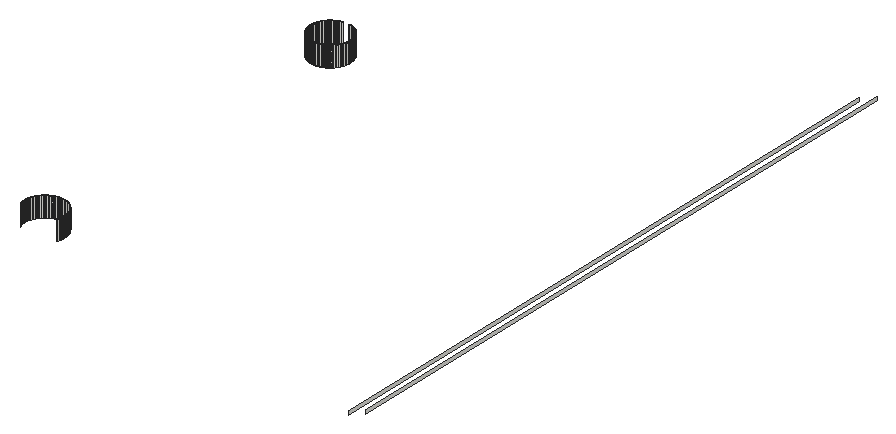
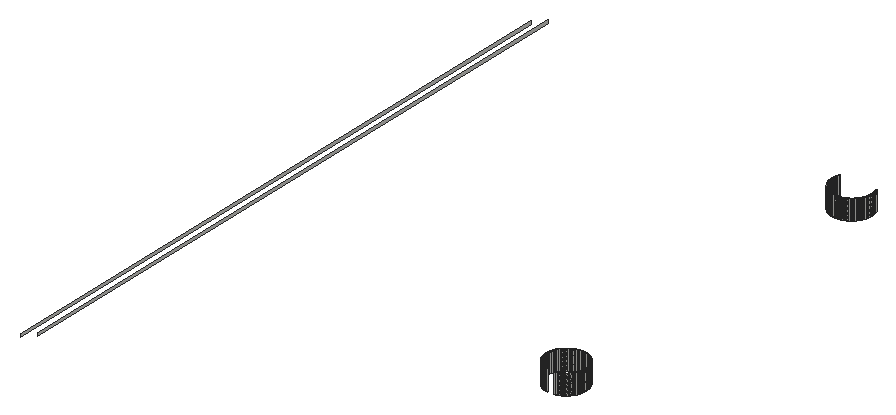
# SketchUp Ruby script. Lengths in inches.
U = 1.inch
M = Sketchup.active_model
def pt(a) = Geom::Point3d.new(a.map { |v| v * U })
def face(e, loops, mat)
  f = e.add_face(loops[0].map { |a| pt(a) })
  loops[1..].each { |l| e.add_face(l.map { |a| pt(a) }).erase! }
  f.material = f.back_material = mat if mat
  f
end
# faces: each face lists its corners as indices into pts; further lists are holes
def faces(e, pts, list, mat = nil) = list.each { |f| face(e, (f[0].is_a?(Array) ? f : [f]).map { |l| l.map { |i| pts[i] } }, mat) }
# xy, xz, yz: faces in a plane at the given z, y or x. An outline is a flat list of corners, or four numbers for a rectangle; further outlines are holes
def ring(l) = l.size == 4 ? [[l[0], l[1]], [l[2], l[1]], [l[2], l[3]], [l[0], l[3]]] : l.each_slice(2).to_a
def flat(e, list, mat, &to3) = list.each { |f| face(e, (f[0].is_a?(Array) ? f : [f]).map { |l| ring(l).map { |u, v| to3.(u, v) } }, mat) }
def xy(e, z, list, mat = nil) = flat(e, list, mat) { |x, y| [x, y, z] }
def xz(e, y, list, mat = nil) = flat(e, list, mat) { |x, z| [x, y, z] }
def yz(e, x, list, mat = nil) = flat(e, list, mat) { |y, z| [x, y, z] }
def lines(e, pts, list) = list.each { |a, b| e.add_line(pt(pts[a]), pt(pts[b])) }
# prism: a flat outline (further loops are holes) pulled along v
def prism(e, loops, v, mat = nil)
  f = face(e, loops, mat); d = Geom::Vector3d.new(v.map { |x| x * U })
  f.pushpull(f.normal.samedirection?(d) ? d.length : -d.length)
end
def box(e, o, s, mat = nil) = prism(e, [[o, [o[0] + s[0], o[1], o[2]], [o[0] + s[0], o[1] + s[1], o[2]], [o[0], o[1] + s[1], o[2]]]], [0, 0, s[2]], mat)
def at(x, y, z, deg = 0) = Geom::Transformation.translation(pt([x, y, z])) * Geom::Transformation.rotation(ORIGIN, Z_AXIS, deg.degrees)
def axes(o, x, y, z) = Geom::Transformation.new([*x, 0, *y, 0, *z, 0, *pt(o).to_a, 1])
def part(name) = M.definitions.add(name)
# library, detail: a bought-in or finely detailed component or shape, given as its bounding box
def library(name, o, s) = part(name).tap { |d| box(d.entities, o, s) }
def detail(e, o, s) = box(e.add_group.entities, o, s)
def put(e, d, t, mat = nil) = e.add_instance(d, t).tap { |i| i.material = mat if mat }
def group(e, t, mat = nil) = e.add_group.tap { |g| g.transformation = t; g.material = mat if mat }.entities
root = M.entities
xz(root,178.75,[[100.84,129,100.92,132],[100.92,129,101,132],[101,129,101.08,132],[101.08,129,101.16,132]])
xz(root,226.5,[[100.84,129,100.92,132],[100.92,129,101,132],[101,129,101.08,132],[101.08,129,101.16,132]])
yz(root,98,[[175.59,129,175.67,132],[175.75,129,175.83,132],[175.83,129,175.91,132],[229.34,129,229.42,132],[229.42,129,229.5,132],
  [229.5,129,229.58,132],[229.58,129,229.66,132]])
yz(root,104,[[175.59,129,175.67,132],[175.67,129,175.75,132],[175.75,129,175.83,132],[175.83,129,175.91,132],[229.34,129,229.42,132],
  [229.42,129,229.5,132],[229.5,129,229.58,132],[229.58,129,229.66,132]])
yz(root,156.5,[[163.5,129,259.5,129.5]])
yz(root,158,[[165,129,261,129.5]])
p = [[98.23,174.6,129],[98.2,174.67,129],[98.2,174.67,132],[98.23,174.6,132],[103.8,174.67,129],[103.77,174.6,129],
  [103.77,174.6,132],[103.8,174.67,132],[98.17,174.75,129],[98.15,174.82,129],[98.15,174.82,132],[98.17,174.75,132],
  [103.83,174.75,129],[103.83,174.75,132],[103.85,174.82,129],[103.85,174.82,132],[98.125,174.9,129],[98.125,174.9,132],
  [103.875,174.9,129],[103.875,174.9,132],[98.1,174.97,129],[98.1,174.97,132],[103.9,174.97,129],[103.9,174.97,132],
  [98.08,175.05,129],[98.07,175.125,129],[98.07,175.125,132],[98.08,175.05,132],[103.92,175.05,129],[103.92,175.05,132],
  [103.93,175.125,129],[103.93,175.125,132],[98.05,175.2,129],[98.05,175.2,132],[103.95,175.2,129],[103.95,175.2,132],
  [98.04,175.28,129],[98.04,175.28,132],[103.96,175.28,129],[103.96,175.28,132],[98.03,175.36,129],[98.03,175.36,132],
  [103.97,175.36,129],[103.97,175.36,132],[98.02,175.4375,129],[98.01,175.51,129],[98.01,175.51,132],[98.02,175.4375,132],
  [103.98,175.4375,129],[103.98,175.4375,132],[103.99,175.51,129],[103.99,175.51,132],[98,175.59,129],[98,175.59,132],
  [104,175.59,129],[104,175.59,132],[98,175.91,129],[98.01,175.99,129],[98.01,175.99,132],[98,175.91,132],
  [103.99,175.99,129],[104,175.91,129],[104,175.91,132],[103.99,175.99,132],[98.02,176.0625,129],[98.02,176.0625,132],
  [103.98,176.0625,129],[103.98,176.0625,132],[98.03,176.14,129],[98.03,176.14,132],[98.04,176.22,129],[98.04,176.22,132],
  [103.96,176.22,129],[103.97,176.14,129],[103.97,176.14,132],[103.96,176.22,132],[98.05,176.3,129],[98.05,176.3,132],
  [103.95,176.3,129],[103.95,176.3,132],[98.07,176.375,129],[98.07,176.375,132],[103.93,176.375,129],[103.93,176.375,132],
  [98.08,176.45,129],[98.08,176.45,132],[103.92,176.45,129],[103.92,176.45,132],[98.1,176.53,129],[98.1,176.53,132],
  [98.125,176.6,129],[98.125,176.6,132],[103.875,176.6,129],[103.9,176.53,129],[103.9,176.53,132],[103.875,176.6,132],
  [98.15,176.68,129],[98.15,176.68,132],[103.85,176.68,129],[103.85,176.68,132],[98.17,176.75,129],[98.17,176.75,132],
  [103.83,176.75,129],[103.83,176.75,132],[98.2,176.83,129],[98.2,176.83,132],[98.23,176.9,129],[98.23,176.9,132],
  [103.77,176.9,129],[103.8,176.83,129],[103.8,176.83,132],[103.77,176.9,132],[98.26,176.97,129],[98.26,176.97,132],
  [103.74,176.97,129],[103.74,176.97,132],[98.29,177.04,129],[98.29,177.04,132],[98.33,177.11,129],[98.33,177.11,132],
  [103.67,177.11,129],[103.71,177.04,129],[103.71,177.04,132],[103.67,177.11,132],[98.36,177.18,129],[98.36,177.18,132],
  [103.64,177.18,129],[103.64,177.18,132],[98.4,177.25,129],[98.4,177.25,132],[98.44,177.32,129],[98.44,177.32,132],
  [103.56,177.32,129],[103.6,177.25,129],[103.6,177.25,132],[103.56,177.32,132],[98.48,177.38,129],[98.48,177.38,132],
  [103.52,177.38,129],[103.52,177.38,132],[98.53,177.45,129],[98.53,177.45,132],[98.57,177.51,129],[98.57,177.51,132],
  [103.43,177.51,129],[103.47,177.45,129],[103.47,177.45,132],[103.43,177.51,132],[98.62,177.58,129],[98.62,177.58,132],
  [103.38,177.58,129],[103.38,177.58,132],[98.67,177.64,129],[98.67,177.64,132],[98.72,177.7,129],[98.72,177.7,132],
  [103.28,177.7,129],[103.33,177.64,129],[103.33,177.64,132],[103.28,177.7,132],[98.77,177.76,129],[98.77,177.76,132],
  [103.23,177.76,129],[103.23,177.76,132],[98.82,177.82,129],[98.82,177.82,132],[98.88,177.87,129],[98.88,177.87,132],
  [103.12,177.87,129],[103.18,177.82,129],[103.18,177.82,132],[103.12,177.87,132],[98.93,177.93,129],[98.93,177.93,132],
  [98.99,177.98,129],[98.99,177.98,132],[103.01,177.98,129],[103.07,177.93,129],[103.07,177.93,132],[103.01,177.98,132],
  [99.05,178.03,129],[99.05,178.03,132],[99.11,178.08,129],[99.11,178.08,132],[102.89,178.08,129],[102.95,178.03,129],
  [102.95,178.03,132],[102.89,178.08,132],[99.17,178.13,129],[99.17,178.13,132],[99.24,178.18,129],[99.24,178.18,132],
  [102.76,178.18,129],[102.83,178.13,129],[102.83,178.13,132],[102.76,178.18,132],[99.3,178.22,129],[99.3,178.22,132],
  [99.37,178.27,129],[99.37,178.27,132],[102.63,178.27,129],[102.7,178.22,129],[102.7,178.22,132],[102.63,178.27,132],
  [99.43,178.31,129],[99.43,178.31,132],[99.5,178.35,129],[99.5,178.35,132],[99.57,178.39,129],[99.57,178.39,132],
  [102.43,178.39,129],[102.5,178.35,129],[102.5,178.35,132],[102.43,178.39,132],[102.57,178.31,129],[102.57,178.31,132],
  [99.64,178.42,129],[99.64,178.42,132],[99.71,178.46,129],[99.71,178.46,132],[102.29,178.46,129],[102.36,178.42,129],
  [102.36,178.42,132],[102.29,178.46,132],[99.78,178.49,129],[99.78,178.49,132],[99.85,178.52,129],[99.85,178.52,132],
  [99.92,178.55,129],[99.92,178.55,132],[102.08,178.55,129],[102.15,178.52,129],[102.15,178.52,132],[102.08,178.55,132],
  [102.22,178.49,129],[102.22,178.49,132],[100,178.58,129],[100,178.58,132],[100.07,178.6,129],[100.07,178.6,132],
  [100.15,178.625,129],[100.15,178.625,132],[100.22,178.65,129],[100.22,178.65,132],[100.3,178.67,129],[100.3,178.67,132],
  [101.7,178.67,129],[101.78,178.65,129],[101.78,178.65,132],[101.7,178.67,132],[101.85,178.625,129],[101.85,178.625,132],
  [101.93,178.6,129],[101.93,178.6,132],[102,178.58,129],[102,178.58,132],[100.375,178.68,129],[100.375,178.68,132],
  [100.45,178.7,129],[100.45,178.7,132],[100.53,178.71,129],[100.53,178.71,132],[100.61,178.72,129],[100.61,178.72,132],
  [100.6875,178.73,129],[100.6875,178.73,132],[100.76,178.74,129],[100.76,178.74,132],[100.84,178.75,129],[100.84,178.75,132],
  [101.16,178.75,129],[101.24,178.74,129],[101.24,178.74,132],[101.16,178.75,132],[101.3125,178.73,129],[101.3125,178.73,132],
  [101.39,178.72,129],[101.39,178.72,132],[101.47,178.71,129],[101.47,178.71,132],[101.55,178.7,129],[101.55,178.7,132],
  [101.625,178.68,129],[101.625,178.68,132],[100.53,226.54,129],[100.45,226.55,129],[100.45,226.55,132],[100.53,226.54,132],
  [100.61,226.53,129],[100.61,226.53,132],[100.6875,226.52,129],[100.6875,226.52,132],[100.76,226.51,129],[100.76,226.51,132],
  [100.84,226.5,129],[100.84,226.5,132],[101.24,226.51,129],[101.16,226.5,129],[101.16,226.5,132],[101.24,226.51,132],
  [101.3125,226.52,129],[101.3125,226.52,132],[101.39,226.53,129],[101.39,226.53,132],[101.47,226.54,129],[101.47,226.54,132],
  [101.55,226.55,129],[101.55,226.55,132],[100.07,226.65,129],[100,226.67,129],[100,226.67,132],[100.07,226.65,132],
  [100.15,226.625,129],[100.15,226.625,132],[100.22,226.6,129],[100.22,226.6,132],[100.3,226.58,129],[100.3,226.58,132],
  [100.375,226.57,129],[100.375,226.57,132],[101.625,226.57,129],[101.625,226.57,132],[101.7,226.58,129],[101.7,226.58,132],
  [101.78,226.6,129],[101.78,226.6,132],[101.85,226.625,129],[101.85,226.625,132],[101.93,226.65,129],[101.93,226.65,132],
  [102,226.67,129],[102,226.67,132],[99.85,226.73,129],[99.78,226.76,129],[99.78,226.76,132],[99.85,226.73,132],
  [99.92,226.7,129],[99.92,226.7,132],[102.08,226.7,129],[102.08,226.7,132],[102.15,226.73,129],[102.15,226.73,132],
  [102.22,226.76,129],[102.22,226.76,132],[99.64,226.83,129],[99.57,226.86,129],[99.57,226.86,132],[99.64,226.83,132],
  [99.71,226.79,129],[99.71,226.79,132],[102.29,226.79,129],[102.29,226.79,132],[102.36,226.83,129],[102.36,226.83,132],
  [102.43,226.86,129],[102.43,226.86,132],[99.43,226.94,129],[99.37,226.98,129],[99.37,226.98,132],[99.43,226.94,132],
  [99.5,226.9,129],[99.5,226.9,132],[102.5,226.9,129],[102.5,226.9,132],[102.57,226.94,129],[102.57,226.94,132],
  [102.63,226.98,129],[102.63,226.98,132],[99.3,227.03,129],[99.24,227.07,129],[99.24,227.07,132],[99.3,227.03,132],
  [102.7,227.03,129],[102.7,227.03,132],[102.76,227.07,129],[102.76,227.07,132],[99.17,227.12,129],[99.11,227.17,129],
  [99.11,227.17,132],[99.17,227.12,132],[102.83,227.12,129],[102.83,227.12,132],[102.89,227.17,129],[102.89,227.17,132],
  [99.05,227.22,129],[98.99,227.27,129],[98.99,227.27,132],[99.05,227.22,132],[102.95,227.22,129],[102.95,227.22,132],
  [103.01,227.27,129],[103.01,227.27,132],[98.93,227.32,129],[98.88,227.38,129],[98.88,227.38,132],[98.93,227.32,132],
  [103.07,227.32,129],[103.07,227.32,132],[103.12,227.38,129],[103.12,227.38,132],[98.82,227.43,129],[98.77,227.49,129],
  [98.77,227.49,132],[98.82,227.43,132],[103.18,227.43,129],[103.18,227.43,132],[103.23,227.49,129],[103.23,227.49,132],
  [98.72,227.55,129],[98.72,227.55,132],[103.28,227.55,129],[103.28,227.55,132],[98.67,227.61,129],[98.62,227.67,129],
  [98.62,227.67,132],[98.67,227.61,132],[103.33,227.61,129],[103.33,227.61,132],[103.38,227.67,129],[103.38,227.67,132],
  [98.57,227.74,129],[98.53,227.8,129],[98.53,227.8,132],[98.57,227.74,132],[103.43,227.74,129],[103.43,227.74,132],
  [103.47,227.8,129],[103.47,227.8,132],[98.48,227.87,129],[98.48,227.87,132],[103.52,227.87,129],[103.52,227.87,132],
  [98.44,227.93,129],[98.4,228,129],[98.4,228,132],[98.44,227.93,132],[103.56,227.93,129],[103.56,227.93,132],
  [103.6,228,129],[103.6,228,132],[98.36,228.07,129],[98.36,228.07,132],[103.64,228.07,129],[103.64,228.07,132],
  [98.33,228.14,129],[98.29,228.21,129],[98.29,228.21,132],[98.33,228.14,132],[103.67,228.14,129],[103.67,228.14,132],
  [103.71,228.21,129],[103.71,228.21,132],[98.26,228.28,129],[98.26,228.28,132],[103.74,228.28,129],[103.74,228.28,132],
  [98.23,228.35,129],[98.23,228.35,132],[103.77,228.35,129],[103.77,228.35,132],[98.2,228.42,129],[98.17,228.5,129],
  [98.17,228.5,132],[98.2,228.42,132],[103.8,228.42,129],[103.8,228.42,132],[103.83,228.5,129],[103.83,228.5,132],
  [98.15,228.57,129],[98.15,228.57,132],[103.85,228.57,129],[103.85,228.57,132],[98.125,228.65,129],[98.1,228.72,129],
  [98.1,228.72,132],[98.125,228.65,132],[103.875,228.65,129],[103.875,228.65,132],[103.9,228.72,129],[103.9,228.72,132],
  [98.08,228.8,129],[98.08,228.8,132],[103.92,228.8,129],[103.92,228.8,132],[98.07,228.875,129],[98.07,228.875,132],
  [103.93,228.875,129],[103.93,228.875,132],[98.05,228.95,129],[98.05,228.95,132],[103.95,228.95,129],[103.95,228.95,132],
  [98.04,229.03,129],[98.03,229.11,129],[98.03,229.11,132],[98.04,229.03,132],[103.96,229.03,129],[103.96,229.03,132],
  [103.97,229.11,129],[103.97,229.11,132],[98.02,229.1875,129],[98.02,229.1875,132],[103.98,229.1875,129],[103.98,229.1875,132],
  [98.01,229.26,129],[98.01,229.26,132],[103.99,229.26,129],[103.99,229.26,132],[98,229.34,129],[98,229.34,132],
  [104,229.34,129],[104,229.34,132],[98,229.66,129],[98.01,229.74,129],[98.01,229.74,132],[98,229.66,132],
  [98.02,229.8125,129],[98.02,229.8125,132],[103.98,229.8125,129],[103.99,229.74,129],[103.99,229.74,132],[103.98,229.8125,132],
  [104,229.66,129],[104,229.66,132],[98.03,229.89,129],[98.03,229.89,132],[103.97,229.89,129],[103.97,229.89,132],
  [98.04,229.97,129],[98.04,229.97,132],[103.96,229.97,129],[103.96,229.97,132],[98.05,230.05,129],[98.05,230.05,132],
  [98.07,230.125,129],[98.07,230.125,132],[103.93,230.125,129],[103.95,230.05,129],[103.95,230.05,132],[103.93,230.125,132],
  [98.08,230.2,129],[98.08,230.2,132],[103.92,230.2,129],[103.92,230.2,132],[98.1,230.28,129],[98.1,230.28,132],
  [103.9,230.28,129],[103.9,230.28,132],[98.125,230.35,129],[98.125,230.35,132],[103.875,230.35,129],[103.875,230.35,132],
  [98.15,230.43,129],[98.15,230.43,132],[98.17,230.5,129],[98.17,230.5,132],[103.83,230.5,129],[103.85,230.43,129],
  [103.85,230.43,132],[103.83,230.5,132],[98.2,230.58,129],[98.2,230.58,132],[103.8,230.58,129],[103.8,230.58,132],
  [98.23,230.65,129],[98.23,230.65,132],[98.26,230.72,129],[98.26,230.72,132],[103.74,230.72,129],[103.77,230.65,129],
  [103.77,230.65,132],[103.74,230.72,132],[98.29,230.79,129],[98.29,230.79,132],[103.71,230.79,129],[103.71,230.79,132],
  [98.33,230.86,129],[98.33,230.86,132],[103.67,230.86,129],[103.67,230.86,132],[98.36,230.93,129],[98.36,230.93,132],
  [98.4,231,129],[98.4,231,132],[103.6,231,129],[103.64,230.93,129],[103.64,230.93,132],[103.6,231,132],
  [98.44,231.07,129],[98.44,231.07,132],[103.56,231.07,129],[103.56,231.07,132],[98.48,231.13,129],[98.48,231.13,132],
  [98.53,231.2,129],[98.53,231.2,132],[103.47,231.2,129],[103.52,231.13,129],[103.52,231.13,132],[103.47,231.2,132],
  [98.57,231.26,129],[98.57,231.26,132],[103.43,231.26,129],[103.43,231.26,132],[98.62,231.33,129],[98.62,231.33,132],
  [98.67,231.39,129],[98.67,231.39,132],[103.33,231.39,129],[103.38,231.33,129],[103.38,231.33,132],[103.33,231.39,132],
  [98.72,231.45,129],[98.72,231.45,132],[98.77,231.51,129],[98.77,231.51,132],[103.23,231.51,129],[103.28,231.45,129],
  [103.28,231.45,132],[103.23,231.51,132],[98.82,231.57,129],[98.82,231.57,132],[103.18,231.57,129],[103.18,231.57,132],
  [98.88,231.62,129],[98.88,231.62,132],[98.93,231.68,129],[98.93,231.68,132],[103.07,231.68,129],[103.12,231.62,129],
  [103.12,231.62,132],[103.07,231.68,132],[98.99,231.73,129],[98.99,231.73,132],[99.05,231.78,129],[99.05,231.78,132],
  [102.95,231.78,129],[103.01,231.73,129],[103.01,231.73,132],[102.95,231.78,132],[99.11,231.83,129],[99.11,231.83,132],
  [99.17,231.88,129],[99.17,231.88,132],[102.83,231.88,129],[102.89,231.83,129],[102.89,231.83,132],[102.83,231.88,132],
  [99.24,231.93,129],[99.24,231.93,132],[99.3,231.97,129],[99.3,231.97,132],[102.7,231.97,129],[102.76,231.93,129],
  [102.76,231.93,132],[102.7,231.97,132],[99.37,232.02,129],[99.37,232.02,132],[99.43,232.06,129],[99.43,232.06,132],
  [102.57,232.06,129],[102.63,232.02,129],[102.63,232.02,132],[102.57,232.06,132],[99.5,232.1,129],[99.5,232.1,132],
  [99.57,232.14,129],[99.57,232.14,132],[99.64,232.17,129],[99.64,232.17,132],[102.36,232.17,129],[102.43,232.14,129],
  [102.43,232.14,132],[102.36,232.17,132],[102.5,232.1,129],[102.5,232.1,132],[99.71,232.21,129],[99.71,232.21,132],
  [99.78,232.24,129],[99.78,232.24,132],[99.85,232.27,129],[99.85,232.27,132],[102.15,232.27,129],[102.22,232.24,129],
  [102.22,232.24,132],[102.15,232.27,132],[102.29,232.21,129],[102.29,232.21,132],[99.92,232.3,129],[99.92,232.3,132],
  [100,232.33,129],[100,232.33,132],[100.07,232.35,129],[100.07,232.35,132],[101.93,232.35,129],[102,232.33,129],
  [102,232.33,132],[101.93,232.35,132],[102.08,232.3,129],[102.08,232.3,132],[100.15,232.375,129],[100.15,232.375,132],
  [100.22,232.4,129],[100.22,232.4,132],[100.3,232.42,129],[100.3,232.42,132],[100.375,232.43,129],[100.375,232.43,132],
  [100.45,232.45,129],[100.45,232.45,132],[100.53,232.46,129],[100.53,232.46,132],[101.47,232.46,129],[101.55,232.45,129],
  [101.55,232.45,132],[101.47,232.46,132],[101.625,232.43,129],[101.625,232.43,132],[101.7,232.42,129],[101.7,232.42,132],
  [101.78,232.4,129],[101.78,232.4,132],[101.85,232.375,129],[101.85,232.375,132]]
faces(root,p,[[0,1,2,3],[4,5,6,7],[8,9,10,11],[1,8,11,2],[12,4,7,13],[14,12,13,15],[9,16,17,10],[18,14,15,19],
  [16,20,21,17],[22,18,19,23],[24,25,26,27],[20,24,27,21],[28,22,23,29],[30,28,29,31],[25,32,33,26],[34,30,31,35],
  [32,36,37,33],[38,34,35,39],[36,40,41,37],[42,38,39,43],[44,45,46,47],[40,44,47,41],[48,42,43,49],[50,48,49,51],
  [45,52,53,46],[54,50,51,55],[56,57,58,59],[60,61,62,63],[57,64,65,58],[66,60,63,67],[64,68,69,65],[68,70,71,69],
  [72,73,74,75],[73,66,67,74],[70,76,77,71],[78,72,75,79],[76,80,81,77],[82,78,79,83],[80,84,85,81],[86,82,83,87],
  [84,88,89,85],[88,90,91,89],[92,93,94,95],[93,86,87,94],[90,96,97,91],[98,92,95,99],[96,100,101,97],[102,98,99,103],
  [100,104,105,101],[104,106,107,105],[108,109,110,111],[109,102,103,110],[106,112,113,107],[114,108,111,115],[112,116,117,113],[116,118,119,117],
  [120,121,122,123],[121,114,115,122],[118,124,125,119],[126,120,123,127],[124,128,129,125],[128,130,131,129],[132,133,134,135],[133,126,127,134],
  [130,136,137,131],[138,132,135,139],[136,140,141,137],[140,142,143,141],[144,145,146,147],[145,138,139,146],[142,148,149,143],[150,144,147,151],
  [148,152,153,149],[152,154,155,153],[156,157,158,159],[157,150,151,158],[154,160,161,155],[162,156,159,163],[160,164,165,161],[164,166,167,165],
  [168,169,170,171],[169,162,163,170],[166,172,173,167],[172,174,175,173],[176,177,178,179],[177,168,171,178],[174,180,181,175],[180,182,183,181],
  [184,185,186,187],[185,176,179,186],[182,188,189,183],[188,190,191,189],[192,193,194,195],[193,184,187,194],[190,196,197,191],[196,198,199,197],
  [200,201,202,203],[201,192,195,202],[198,204,205,199],[204,206,207,205],[206,208,209,207],[210,211,212,213],[211,214,215,212],[214,200,203,215],
  [208,216,217,209],[216,218,219,217],[220,221,222,223],[221,210,213,222],[218,224,225,219],[224,226,227,225],[226,228,229,227],[230,231,232,233],
  [231,234,235,232],[234,220,223,235],[228,236,237,229],[236,238,239,237],[238,240,241,239],[240,242,243,241],[242,244,245,243],[246,247,248,249],
  [247,250,251,248],[250,252,253,251],[252,254,255,253],[254,230,233,255],[244,256,257,245],[256,258,259,257],[258,260,261,259],[260,262,263,261],
  [262,264,265,263],[264,266,267,265],[266,268,269,267],[270,271,272,273],[271,274,275,272],[274,276,277,275],[276,278,279,277],[278,280,281,279],
  [280,282,283,281],[282,246,249,283],[284,285,286,287],[288,284,287,289],[290,288,289,291],[292,290,291,293],[294,292,293,295],[296,297,298,299],
  [300,296,299,301],[302,300,301,303],[304,302,303,305],[306,304,305,307],[308,309,310,311],[312,308,311,313],[314,312,313,315],[316,314,315,317],
  [318,316,317,319],[285,318,319,286],[320,306,307,321],[322,320,321,323],[324,322,323,325],[326,324,325,327],[328,326,327,329],[330,328,329,331],
  [332,333,334,335],[336,332,335,337],[309,336,337,310],[338,330,331,339],[340,338,339,341],[342,340,341,343],[344,345,346,347],[348,344,347,349],
  [333,348,349,334],[350,342,343,351],[352,350,351,353],[354,352,353,355],[356,357,358,359],[360,356,359,361],[345,360,361,346],[362,354,355,363],
  [364,362,363,365],[366,364,365,367],[368,369,370,371],[357,368,371,358],[372,366,367,373],[374,372,373,375],[376,377,378,379],[369,376,379,370],
  [380,374,375,381],[382,380,381,383],[384,385,386,387],[377,384,387,378],[388,382,383,389],[390,388,389,391],[392,393,394,395],[385,392,395,386],
  [396,390,391,397],[398,396,397,399],[400,401,402,403],[393,400,403,394],[404,398,399,405],[406,404,405,407],[401,408,409,402],[410,406,407,411],
  [412,413,414,415],[408,412,415,409],[416,410,411,417],[418,416,417,419],[420,421,422,423],[413,420,423,414],[424,418,419,425],[426,424,425,427],
  [421,428,429,422],[430,426,427,431],[432,433,434,435],[428,432,435,429],[436,430,431,437],[438,436,437,439],[433,440,441,434],[442,438,439,443],
  [444,445,446,447],[440,444,447,441],[448,442,443,449],[450,448,449,451],[445,452,453,446],[454,450,451,455],[452,456,457,453],[458,454,455,459],
  [460,461,462,463],[456,460,463,457],[464,458,459,465],[466,464,465,467],[461,468,469,462],[470,466,467,471],[472,473,474,475],[468,472,475,469],
  [476,470,471,477],[478,476,477,479],[473,480,481,474],[482,478,479,483],[480,484,485,481],[486,482,483,487],[484,488,489,485],[490,486,487,491],
  [492,493,494,495],[488,492,495,489],[496,490,491,497],[498,496,497,499],[493,500,501,494],[502,498,499,503],[500,504,505,501],[506,502,503,507],
  [504,508,509,505],[510,506,507,511],[512,513,514,515],[513,516,517,514],[518,519,520,521],[519,522,523,520],[516,524,525,517],[526,518,521,527],
  [524,528,529,525],[530,526,527,531],[528,532,533,529],[532,534,535,533],[536,537,538,539],[537,530,531,538],[534,540,541,535],[542,536,539,543],
  [540,544,545,541],[546,542,543,547],[544,548,549,545],[550,546,547,551],[548,552,553,549],[552,554,555,553],[556,557,558,559],[557,550,551,558],
  [554,560,561,555],[562,556,559,563],[560,564,565,561],[564,566,567,565],[568,569,570,571],[569,562,563,570],[566,572,573,567],[574,568,571,575],
  [572,576,577,573],[578,574,575,579],[576,580,581,577],[580,582,583,581],[584,585,586,587],[585,578,579,586],[582,588,589,583],[590,584,587,591],
  [588,592,593,589],[592,594,595,593],[596,597,598,599],[597,590,591,598],[594,600,601,595],[602,596,599,603],[600,604,605,601],[604,606,607,605],
  [608,609,610,611],[609,602,603,610],[606,612,613,607],[612,614,615,613],[616,617,618,619],[617,608,611,618],[614,620,621,615],[622,616,619,623],
  [620,624,625,621],[624,626,627,625],[628,629,630,631],[629,622,623,630],[626,632,633,627],[632,634,635,633],[636,637,638,639],[637,628,631,638],
  [634,640,641,635],[640,642,643,641],[644,645,646,647],[645,636,639,646],[642,648,649,643],[648,650,651,649],[652,653,654,655],[653,644,647,654],
  [650,656,657,651],[656,658,659,657],[660,661,662,663],[661,652,655,662],[658,664,665,659],[664,666,667,665],[666,668,669,667],[670,671,672,673],
  [671,674,675,672],[674,660,663,675],[668,676,677,669],[676,678,679,677],[678,680,681,679],[682,683,684,685],[683,686,687,684],[686,670,673,687],
  [680,688,689,681],[688,690,691,689],[690,692,693,691],[694,695,696,697],[695,698,699,696],[698,682,685,699],[692,700,701,693],[700,702,703,701],
  [702,704,705,703],[704,706,707,705],[706,708,709,707],[708,710,711,709],[712,713,714,715],[713,716,717,714],[716,718,719,717],[718,720,721,719],
  [720,722,723,721],[722,694,697,723]])
